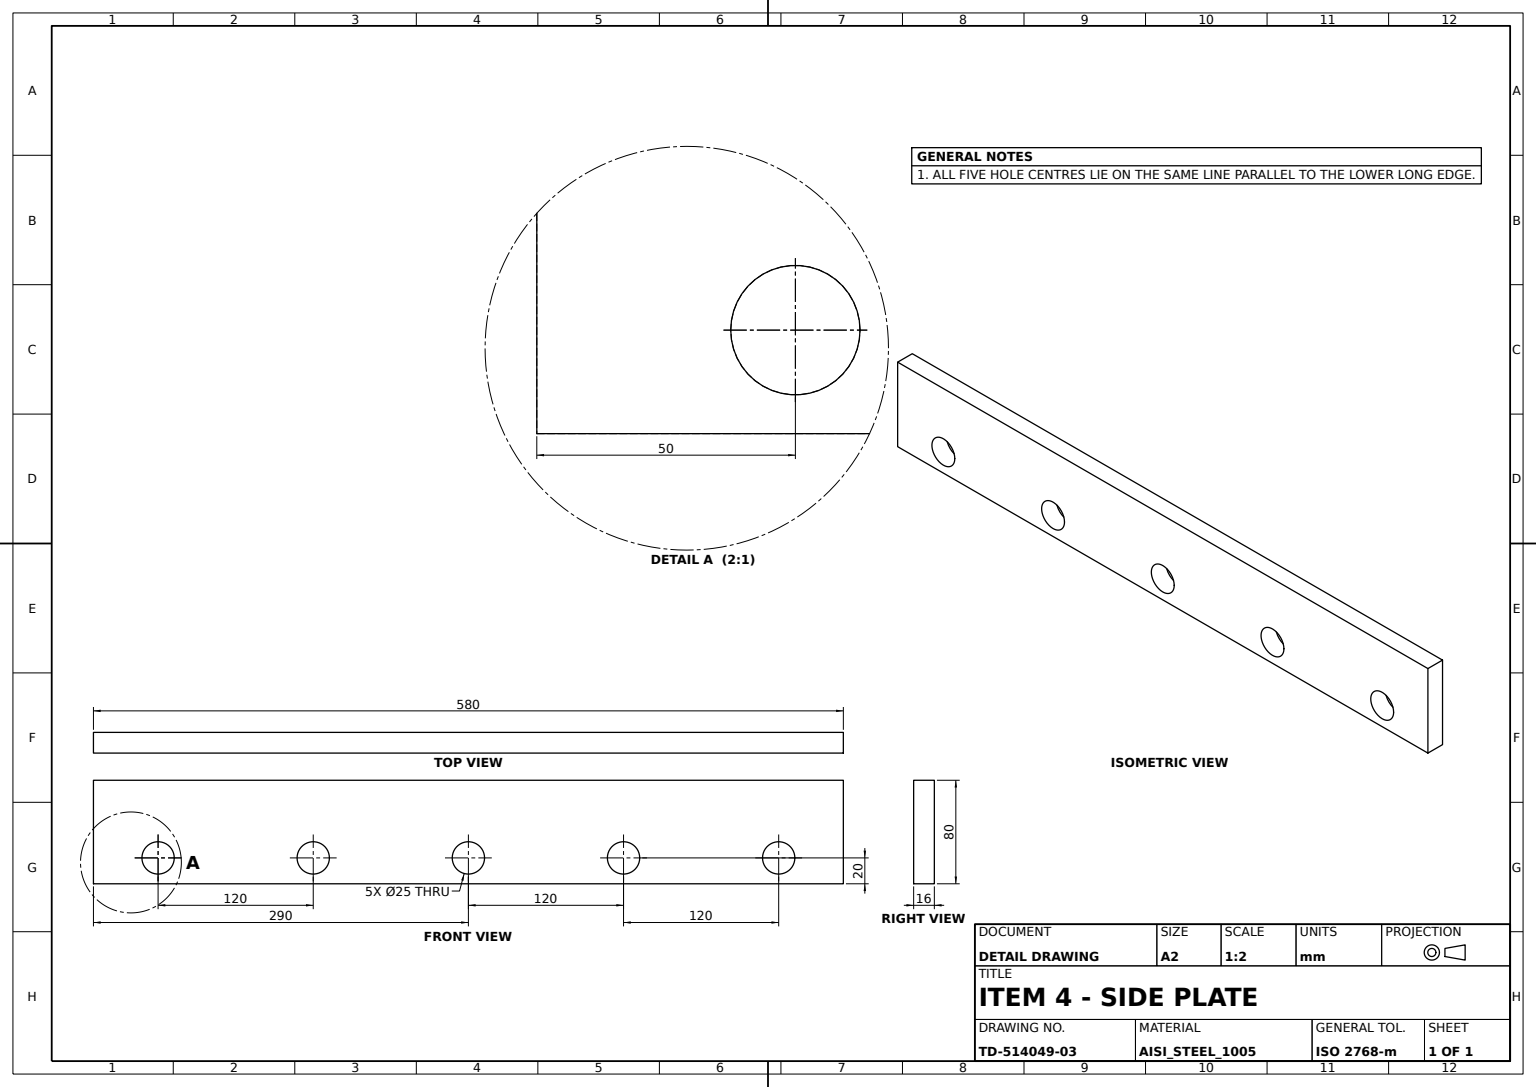
ISO-10303-21;
HEADER;
FILE_DESCRIPTION((''),'2;1');
FILE_NAME('','',(''),(''),'','','');
FILE_SCHEMA(('AUTOMOTIVE_DESIGN'));
ENDSEC;
DATA;
#1=APPLICATION_CONTEXT('');
#2=PRODUCT_CONTEXT('',#1,'mechanical');
#3=PRODUCT('','','',(#2));
#4=PRODUCT_DEFINITION_FORMATION('','',#3);
#5=PRODUCT_DEFINITION_CONTEXT('',#1,'design');
#6=PRODUCT_DEFINITION('','',#4,#5);
#7=PRODUCT_DEFINITION_SHAPE('','',#6);
#8=(LENGTH_UNIT()NAMED_UNIT(*)SI_UNIT(.MILLI.,.METRE.));
#9=(NAMED_UNIT(*)PLANE_ANGLE_UNIT()SI_UNIT($,.RADIAN.));
#10=(NAMED_UNIT(*)SI_UNIT($,.STERADIAN.)SOLID_ANGLE_UNIT());
#11=UNCERTAINTY_MEASURE_WITH_UNIT(LENGTH_MEASURE(0.005),#8,'distance_accuracy_value','');
#12=(GEOMETRIC_REPRESENTATION_CONTEXT(3)GLOBAL_UNCERTAINTY_ASSIGNED_CONTEXT((#11))GLOBAL_UNIT_ASSIGNED_CONTEXT((#8,#9,#10))REPRESENTATION_CONTEXT('',''));
#13=CARTESIAN_POINT('',(-290.,80.,16.));
#14=VERTEX_POINT('',#13);
#15=CARTESIAN_POINT('',(-290.,80.,0.));
#16=VERTEX_POINT('',#15);
#17=DIRECTION('',(0.,0.,-1.));
#18=VECTOR('',#17,1000.);
#19=LINE('',#13,#18);
#20=EDGE_CURVE('',#14,#16,#19,.T.);
#21=ORIENTED_EDGE('',*,*,#20,.T.);
#22=CARTESIAN_POINT('',(-290.,0.,0.));
#23=VERTEX_POINT('',#22);
#24=DIRECTION('',(0.,-1.,0.));
#25=VECTOR('',#24,1000.);
#26=LINE('',#15,#25);
#27=EDGE_CURVE('',#16,#23,#26,.T.);
#28=ORIENTED_EDGE('',*,*,#27,.T.);
#29=CARTESIAN_POINT('',(-290.,0.,16.));
#30=VERTEX_POINT('',#29);
#31=LINE('',#29,#18);
#32=EDGE_CURVE('',#30,#23,#31,.T.);
#33=ORIENTED_EDGE('',*,*,#32,.F.);
#34=LINE('',#13,#25);
#35=EDGE_CURVE('',#14,#30,#34,.T.);
#36=ORIENTED_EDGE('',*,*,#35,.F.);
#37=EDGE_LOOP('',(#21,#28,#33,#36));
#38=FACE_BOUND('',#37,.T.);
#39=DIRECTION('',(1.,0.,0.));
#40=DIRECTION('',(0.,1.,0.));
#41=AXIS2_PLACEMENT_3D('',#13,#39,#40);
#42=PLANE('',#41);
#43=ADVANCED_FACE('',(#38),#42,.F.);
#44=ORIENTED_EDGE('',*,*,#32,.T.);
#45=CARTESIAN_POINT('',(290.,0.,0.));
#46=VERTEX_POINT('',#45);
#47=VECTOR('',#39,1000.);
#48=LINE('',#22,#47);
#49=EDGE_CURVE('',#23,#46,#48,.T.);
#50=ORIENTED_EDGE('',*,*,#49,.T.);
#51=CARTESIAN_POINT('',(290.,0.,16.));
#52=VERTEX_POINT('',#51);
#53=LINE('',#51,#18);
#54=EDGE_CURVE('',#52,#46,#53,.T.);
#55=ORIENTED_EDGE('',*,*,#54,.F.);
#56=LINE('',#29,#47);
#57=EDGE_CURVE('',#30,#52,#56,.T.);
#58=ORIENTED_EDGE('',*,*,#57,.F.);
#59=EDGE_LOOP('',(#44,#50,#55,#58));
#60=FACE_BOUND('',#59,.T.);
#61=DIRECTION('',(-1.,0.,0.));
#62=AXIS2_PLACEMENT_3D('',#29,#40,#61);
#63=PLANE('',#62);
#64=ADVANCED_FACE('',(#60),#63,.F.);
#65=CARTESIAN_POINT('',(290.,80.,16.));
#66=VERTEX_POINT('',#65);
#67=VECTOR('',#40,1000.);
#68=LINE('',#51,#67);
#69=EDGE_CURVE('',#52,#66,#68,.T.);
#70=ORIENTED_EDGE('',*,*,#69,.T.);
#71=VECTOR('',#61,1000.);
#72=LINE('',#65,#71);
#73=EDGE_CURVE('',#66,#14,#72,.T.);
#74=ORIENTED_EDGE('',*,*,#73,.T.);
#75=ORIENTED_EDGE('',*,*,#35,.T.);
#76=ORIENTED_EDGE('',*,*,#57,.T.);
#77=EDGE_LOOP('',(#70,#74,#75,#76));
#78=FACE_BOUND('',#77,.T.);
#79=CARTESIAN_POINT('',(-107.5,20.,16.));
#80=VERTEX_POINT('',#79);
#81=CARTESIAN_POINT('',(-120.,20.,16.));
#82=DIRECTION('',(0.,0.,1.));
#83=AXIS2_PLACEMENT_3D('',#81,#82,#39);
#84=CIRCLE('',#83,12.5);
#85=EDGE_CURVE('',#80,#80,#84,.T.);
#86=ORIENTED_EDGE('',*,*,#85,.F.);
#87=EDGE_LOOP('',(#86));
#88=FACE_BOUND('',#87,.T.);
#89=CARTESIAN_POINT('',(132.5,20.,16.));
#90=VERTEX_POINT('',#89);
#91=CARTESIAN_POINT('',(120.,20.,16.));
#92=AXIS2_PLACEMENT_3D('',#91,#82,#39);
#93=CIRCLE('',#92,12.5);
#94=EDGE_CURVE('',#90,#90,#93,.T.);
#95=ORIENTED_EDGE('',*,*,#94,.F.);
#96=EDGE_LOOP('',(#95));
#97=FACE_BOUND('',#96,.T.);
#98=CARTESIAN_POINT('',(12.5,20.,16.));
#99=VERTEX_POINT('',#98);
#100=CARTESIAN_POINT('',(0.,20.,16.));
#101=AXIS2_PLACEMENT_3D('',#100,#82,#39);
#102=CIRCLE('',#101,12.5);
#103=EDGE_CURVE('',#99,#99,#102,.T.);
#104=ORIENTED_EDGE('',*,*,#103,.F.);
#105=EDGE_LOOP('',(#104));
#106=FACE_BOUND('',#105,.T.);
#107=CARTESIAN_POINT('',(252.5,20.,16.));
#108=VERTEX_POINT('',#107);
#109=CARTESIAN_POINT('',(240.,20.,16.));
#110=AXIS2_PLACEMENT_3D('',#109,#82,#39);
#111=CIRCLE('',#110,12.5);
#112=EDGE_CURVE('',#108,#108,#111,.T.);
#113=ORIENTED_EDGE('',*,*,#112,.F.);
#114=EDGE_LOOP('',(#113));
#115=FACE_BOUND('',#114,.T.);
#116=CARTESIAN_POINT('',(-227.5,20.,16.));
#117=VERTEX_POINT('',#116);
#118=CARTESIAN_POINT('',(-240.,20.,16.));
#119=AXIS2_PLACEMENT_3D('',#118,#82,#39);
#120=CIRCLE('',#119,12.5);
#121=EDGE_CURVE('',#117,#117,#120,.T.);
#122=ORIENTED_EDGE('',*,*,#121,.F.);
#123=EDGE_LOOP('',(#122));
#124=FACE_BOUND('',#123,.T.);
#125=PLANE('',#119);
#126=ADVANCED_FACE('',(#78,#88,#97,#106,#115,#124),#125,.T.);
#127=ORIENTED_EDGE('',*,*,#112,.T.);
#128=EDGE_LOOP('',(#127));
#129=FACE_BOUND('',#128,.T.);
#130=CARTESIAN_POINT('',(252.5,20.,0.));
#131=VERTEX_POINT('',#130);
#132=CARTESIAN_POINT('',(240.,20.,0.));
#133=AXIS2_PLACEMENT_3D('',#132,#82,#39);
#134=CIRCLE('',#133,12.5);
#135=EDGE_CURVE('',#131,#131,#134,.T.);
#136=ORIENTED_EDGE('',*,*,#135,.F.);
#137=EDGE_LOOP('',(#136));
#138=FACE_BOUND('',#137,.T.);
#139=AXIS2_PLACEMENT_3D('',#109,#17,#61);
#140=CYLINDRICAL_SURFACE('',#139,12.5);
#141=ADVANCED_FACE('',(#129,#138),#140,.F.);
#142=ORIENTED_EDGE('',*,*,#49,.F.);
#143=ORIENTED_EDGE('',*,*,#27,.F.);
#144=CARTESIAN_POINT('',(290.,80.,0.));
#145=VERTEX_POINT('',#144);
#146=LINE('',#144,#71);
#147=EDGE_CURVE('',#145,#16,#146,.T.);
#148=ORIENTED_EDGE('',*,*,#147,.F.);
#149=LINE('',#45,#67);
#150=EDGE_CURVE('',#46,#145,#149,.T.);
#151=ORIENTED_EDGE('',*,*,#150,.F.);
#152=EDGE_LOOP('',(#142,#143,#148,#151));
#153=FACE_BOUND('',#152,.T.);
#154=ORIENTED_EDGE('',*,*,#135,.T.);
#155=EDGE_LOOP('',(#154));
#156=FACE_BOUND('',#155,.T.);
#157=CARTESIAN_POINT('',(-227.5,20.,0.));
#158=VERTEX_POINT('',#157);
#159=CARTESIAN_POINT('',(-240.,20.,0.));
#160=AXIS2_PLACEMENT_3D('',#159,#82,#39);
#161=CIRCLE('',#160,12.5);
#162=EDGE_CURVE('',#158,#158,#161,.T.);
#163=ORIENTED_EDGE('',*,*,#162,.T.);
#164=EDGE_LOOP('',(#163));
#165=FACE_BOUND('',#164,.T.);
#166=CARTESIAN_POINT('',(-107.5,20.,0.));
#167=VERTEX_POINT('',#166);
#168=CARTESIAN_POINT('',(-120.,20.,0.));
#169=AXIS2_PLACEMENT_3D('',#168,#82,#39);
#170=CIRCLE('',#169,12.5);
#171=EDGE_CURVE('',#167,#167,#170,.T.);
#172=ORIENTED_EDGE('',*,*,#171,.T.);
#173=EDGE_LOOP('',(#172));
#174=FACE_BOUND('',#173,.T.);
#175=CARTESIAN_POINT('',(132.5,20.,0.));
#176=VERTEX_POINT('',#175);
#177=CARTESIAN_POINT('',(120.,20.,0.));
#178=AXIS2_PLACEMENT_3D('',#177,#82,#39);
#179=CIRCLE('',#178,12.5);
#180=EDGE_CURVE('',#176,#176,#179,.T.);
#181=ORIENTED_EDGE('',*,*,#180,.T.);
#182=EDGE_LOOP('',(#181));
#183=FACE_BOUND('',#182,.T.);
#184=CARTESIAN_POINT('',(12.5,20.,0.));
#185=VERTEX_POINT('',#184);
#186=CARTESIAN_POINT('',(0.,20.,0.));
#187=AXIS2_PLACEMENT_3D('',#186,#82,#39);
#188=CIRCLE('',#187,12.5);
#189=EDGE_CURVE('',#185,#185,#188,.T.);
#190=ORIENTED_EDGE('',*,*,#189,.T.);
#191=EDGE_LOOP('',(#190));
#192=FACE_BOUND('',#191,.T.);
#193=PLANE('',#160);
#194=ADVANCED_FACE('',(#153,#156,#165,#174,#183,#192),#193,.F.);
#195=ORIENTED_EDGE('',*,*,#103,.T.);
#196=EDGE_LOOP('',(#195));
#197=FACE_BOUND('',#196,.T.);
#198=ORIENTED_EDGE('',*,*,#189,.F.);
#199=EDGE_LOOP('',(#198));
#200=FACE_BOUND('',#199,.T.);
#201=AXIS2_PLACEMENT_3D('',#100,#17,#61);
#202=CYLINDRICAL_SURFACE('',#201,12.5);
#203=ADVANCED_FACE('',(#197,#200),#202,.F.);
#204=ORIENTED_EDGE('',*,*,#54,.T.);
#205=ORIENTED_EDGE('',*,*,#150,.T.);
#206=LINE('',#65,#18);
#207=EDGE_CURVE('',#66,#145,#206,.T.);
#208=ORIENTED_EDGE('',*,*,#207,.F.);
#209=ORIENTED_EDGE('',*,*,#69,.F.);
#210=EDGE_LOOP('',(#204,#205,#208,#209));
#211=FACE_BOUND('',#210,.T.);
#212=AXIS2_PLACEMENT_3D('',#51,#61,#82);
#213=PLANE('',#212);
#214=ADVANCED_FACE('',(#211),#213,.F.);
#215=ORIENTED_EDGE('',*,*,#121,.T.);
#216=EDGE_LOOP('',(#215));
#217=FACE_BOUND('',#216,.T.);
#218=ORIENTED_EDGE('',*,*,#162,.F.);
#219=EDGE_LOOP('',(#218));
#220=FACE_BOUND('',#219,.T.);
#221=AXIS2_PLACEMENT_3D('',#118,#17,#61);
#222=CYLINDRICAL_SURFACE('',#221,12.5);
#223=ADVANCED_FACE('',(#217,#220),#222,.F.);
#224=ORIENTED_EDGE('',*,*,#85,.T.);
#225=EDGE_LOOP('',(#224));
#226=FACE_BOUND('',#225,.T.);
#227=ORIENTED_EDGE('',*,*,#171,.F.);
#228=EDGE_LOOP('',(#227));
#229=FACE_BOUND('',#228,.T.);
#230=AXIS2_PLACEMENT_3D('',#81,#17,#61);
#231=CYLINDRICAL_SURFACE('',#230,12.5);
#232=ADVANCED_FACE('',(#226,#229),#231,.F.);
#233=ORIENTED_EDGE('',*,*,#20,.F.);
#234=ORIENTED_EDGE('',*,*,#73,.F.);
#235=ORIENTED_EDGE('',*,*,#207,.T.);
#236=ORIENTED_EDGE('',*,*,#147,.T.);
#237=EDGE_LOOP('',(#233,#234,#235,#236));
#238=FACE_BOUND('',#237,.T.);
#239=AXIS2_PLACEMENT_3D('',#65,#24,#39);
#240=PLANE('',#239);
#241=ADVANCED_FACE('',(#238),#240,.F.);
#242=ORIENTED_EDGE('',*,*,#180,.F.);
#243=EDGE_LOOP('',(#242));
#244=FACE_BOUND('',#243,.T.);
#245=ORIENTED_EDGE('',*,*,#94,.T.);
#246=EDGE_LOOP('',(#245));
#247=FACE_BOUND('',#246,.T.);
#248=AXIS2_PLACEMENT_3D('',#91,#17,#61);
#249=CYLINDRICAL_SURFACE('',#248,12.5);
#250=ADVANCED_FACE('',(#244,#247),#249,.F.);
#251=CLOSED_SHELL('',(#43,#64,#126,#141,#194,#203,#214,#223,#232,#241,#250));
#252=MANIFOLD_SOLID_BREP('',#251);
#253=ADVANCED_BREP_SHAPE_REPRESENTATION('',(#252),#12);
#254=SHAPE_DEFINITION_REPRESENTATION(#7,#253);
ENDSEC;
END-ISO-10303-21;
